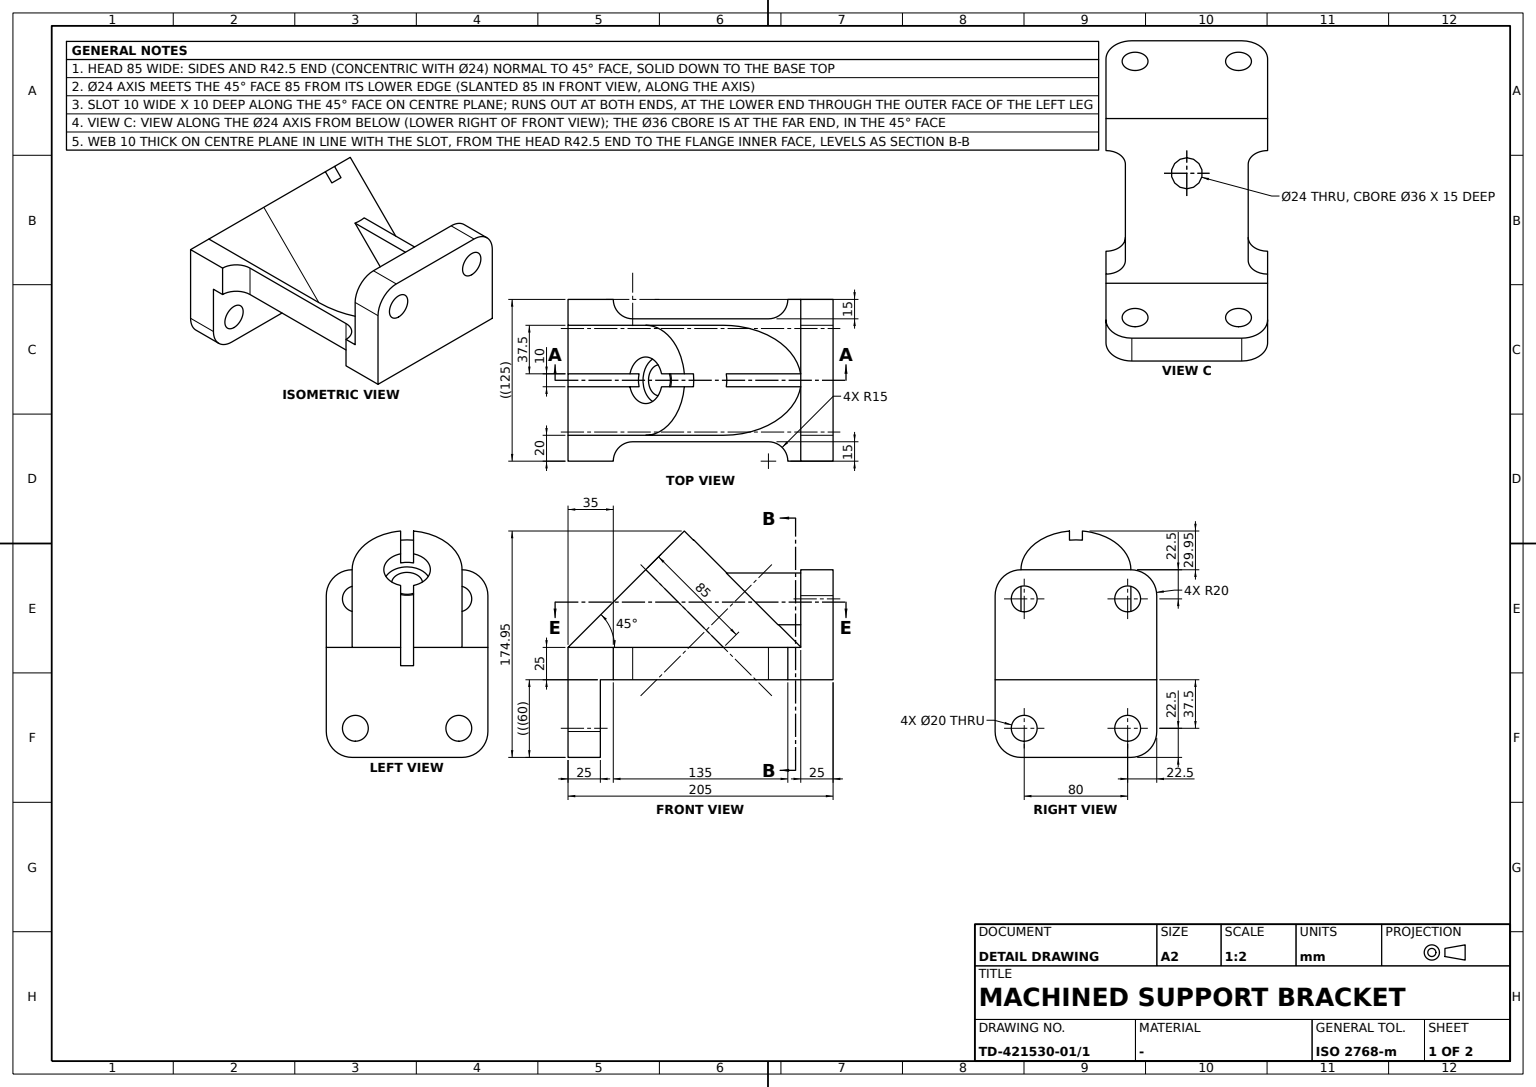
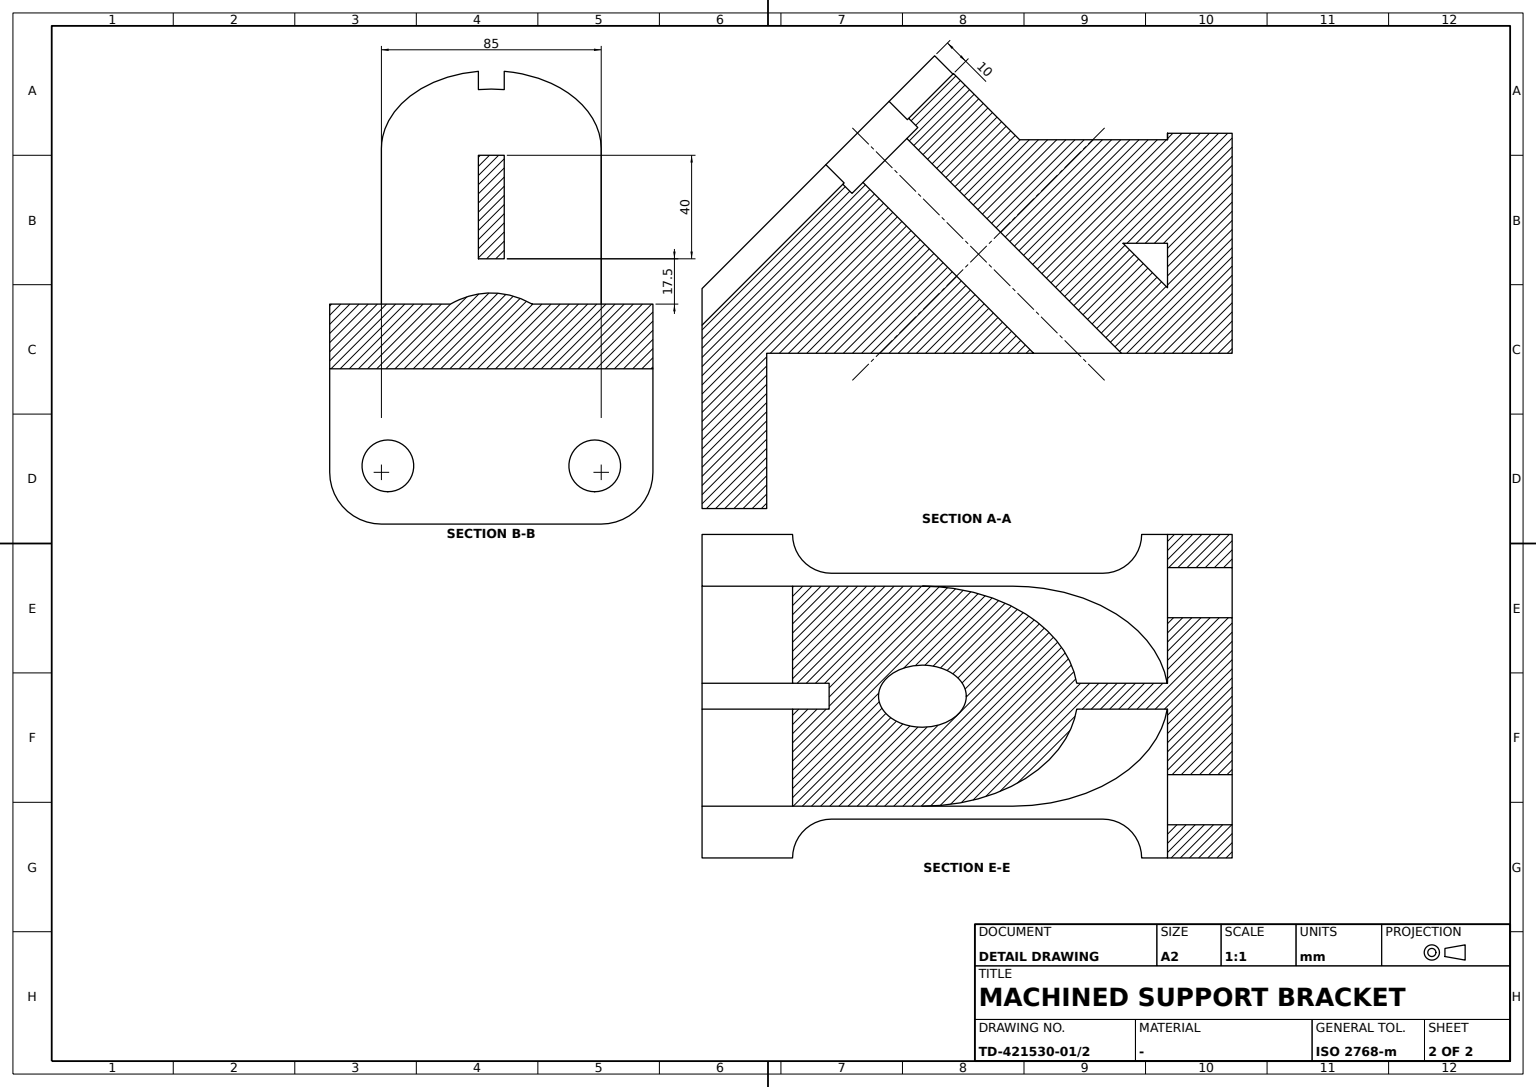
solid
v1 (0,59.678716,-12.5)
e1 v1 v1 ELLIPSE(AX(P(0,42.708153,-12.5),D(0,0,1),D(0,1,0)),16.970563,12) rev
v2 (0,-23.304041,70.482756)
e2 v2 v2 CIRCLE(AX(P(0,-31.789322,61.997475),D(0,0.707106781,-0.707106781),D(0,0.707106781,0.707106781)),12)
face CYL(AX(P(0,-42.325213,72.533366),D(0,0.707106781,-0.707106781),D(1,0,0)),12) rev [e1] [-e2]
v3 (5,77.5,30)
v4 (-5,77.5,30)
e3 v3 v4 LINE
v5 (5,59.894835,30)
e4 v3 v5 LINE
v6 (-5,59.894835,30)
e5 v5 v6 ELLIPSE(AX(P(0,0.208153,30),D(0,0,1),D(0,1,0)),60.104076,42.5)
e6 v4 v6 LINE
face PLANE(AX(P(5,77.5,30),D(0,0,1),D(-1,0,0))) rev [-e3 e4 e5 -e6]
v7 (62.5,67.5,12.5)
v8 (47.5,52.5,12.5)
e7 v7 v8 CIRCLE(AX(P(62.5,52.5,12.5),D(0,0,1),D(1,0,0)),15)
v9 (62.5,77.5,12.5)
e8 v7 v9 LINE
v10 (4.326373,77.5,12.5)
e9 v9 v10 LINE
v11 (42.5,17.708153,12.5)
e10 v11 v10 ELLIPSE(AX(P(0,17.708153,12.5),D(0,0,1),D(0,1,0)),60.104076,42.5)
v12 (42.5,-102.5,12.5)
e11 v12 v11 LINE
v13 (62.5,-102.5,12.5)
e12 v13 v12 LINE
v14 (62.5,-67.5,12.5)
e13 v13 v14 LINE
v15 (47.5,-52.5,12.5)
e14 v15 v14 CIRCLE(AX(P(62.5,-52.5,12.5),D(0,0,1),D(1,0,0)),15)
e15 v8 v15 LINE
face PLANE(AX(P(0,0,12.5),D(0,0,1),D(1,0,0))) [-e7 e8 e9 -e10 -e11 -e12 e13 -e14 -e15]
v16 (-47.5,52.5,-12.5)
v17 (-47.5,52.5,12.5)
e16 v16 v17 LINE
v18 (-62.5,67.5,12.5)
e17 v17 v18 CIRCLE(AX(P(-62.5,52.5,12.5),D(0,0,1),D(1,0,0)),15)
v19 (-62.5,67.5,-12.5)
e18 v19 v18 LINE
e19 v16 v19 CIRCLE(AX(P(-62.5,52.5,-12.5),D(0,0,1),D(1,0,0)),15)
face CYL(AX(P(-62.5,52.5,0),D(0,0,1),D(1,0,0)),15) rev [e16 e17 -e18 -e19]
v20 (47.5,52.5,-12.5)
e20 v20 v8 LINE
v21 (62.5,67.5,-12.5)
e21 v21 v20 CIRCLE(AX(P(62.5,52.5,-12.5),D(0,0,1),D(1,0,0)),15)
e22 v21 v7 LINE
face CYL(AX(P(62.5,52.5,0),D(0,0,1),D(1,0,0)),15) rev [e7 -e20 -e21 e22]
v22 (-40,102.5,40)
e23 v22 v22 CIRCLE(AX(P(-40,102.5,50),D(0,-1,0),D(0,0,-1)),10)
v23 (-62.5,102.5,-12.5)
v24 (-62.5,102.5,52.5)
e24 v23 v24 LINE
v25 (-42.5,102.5,72.5)
e25 v25 v24 CIRCLE(AX(P(-42.5,102.5,52.5),D(0,-1,0),D(0,0,-1)),20)
v26 (42.5,102.5,72.5)
e26 v25 v26 LINE
v27 (62.5,102.5,52.5)
e27 v27 v26 CIRCLE(AX(P(42.5,102.5,52.5),D(0,-1,0),D(0,0,-1)),20)
v28 (62.5,102.5,-12.5)
e28 v28 v27 LINE
e29 v23 v28 LINE
v29 (40,102.5,40)
e30 v29 v29 CIRCLE(AX(P(40,102.5,50),D(0,-1,0),D(0,0,-1)),10)
face PLANE(AX(P(-62.5,102.5,0),D(0,-1,0),D(1,0,0))) rev [e23] [e24 -e25 e26 -e27 -e28 -e29] [e30]
v30 (40,-77.5,-60)
e31 v30 v30 CIRCLE(AX(P(40,-77.5,-50),D(0,-1,0),D(0,0,-1)),10)
v31 (40,-102.5,-40)
e32 v31 v31 CIRCLE(AX(P(40,-102.5,-50),D(0,1,0),D(0,0,1)),10)
face CYL(AX(P(40,0,-50),D(0,1,0),D(-1,0,0)),10) rev [-e31] [-e32]
v32 (5,-5.481515,95.37635)
v33 (5,-23.097837,77.760028)
e33 v32 v33 LINE
v34 (-5,-5.481515,95.37635)
e34 v32 v34 CIRCLE(AX(P(0,-35.324856,65.533009),D(0,-0.707106781,0.707106781),D(0,-0.707106781,-0.707106781)),42.5)
v35 (-5,-23.097837,77.760028)
e35 v35 v34 LINE
e36 v33 v35 CIRCLE(AX(P(0,-35.324856,65.533009),D(0,-0.707106781,0.707106781),D(0,-0.707106781,-0.707106781)),18)
face PLANE(AX(P(0,-50.428932,50.428932),D(0,-0.707106781,0.707106781),D(1,0,0))) [-e33 e34 -e35 -e36]
v36 (0,-19.0614,74.725397)
e37 v36 v36 CIRCLE(AX(P(0,-31.789322,61.997475),D(0,0.707106781,-0.707106781),D(0,0.707106781,0.707106781)),18)
face PLANE(AX(P(12,-31.789322,61.997475),D(0,0.707106781,-0.707106781),D(1,0,0))) rev [-e37] [e2]
v37 (-5,19.894835,70)
v38 (5,19.894835,70)
e38 v37 v38 ELLIPSE(AX(P(0,-39.791847,70),D(0,0,-1),D(0,1,0)),60.104076,42.5)
e39 v6 v37 LINE
e40 v5 v38 LINE
v39 (5,-12.552583,102.447417)
e41 v39 v32 LINE
v40 (42.5,-42.395924,72.604076)
e42 v39 v40 CIRCLE(AX(P(0,-42.395924,72.604076),D(0,0.707106781,-0.707106781),D(0,0.707106781,0.707106781)),42.5)
e43 v40 v11 LINE
v41 (-4.326373,77.5,12.5)
e44 v10 v41 ELLIPSE(AX(P(0,77.5,-47.291847),D(0,1,0),D(0,0,-1)),60.104076,42.5) rev
v42 (-42.5,17.708153,12.5)
e45 v41 v42 ELLIPSE(AX(P(0,17.708153,12.5),D(0,0,1),D(0,1,0)),60.104076,42.5)
v43 (-42.5,-42.395924,72.604076)
e46 v43 v42 LINE
v44 (-5,-12.552583,102.447417)
e47 v43 v44 CIRCLE(AX(P(0,-42.395924,72.604076),D(0,0.707106781,-0.707106781),D(0,0.707106781,0.707106781)),42.5)
e48 v44 v34 LINE
face CYL(AX(P(0,75.695687,-45.487534),D(0,0.707106781,-0.707106781),D(-1,0,0)),42.5) [-e38 -e39 -e5 e40] [-e34 -e41 e42 e43 e10 e44 e45 -e46 e47 e48]
e49 v12 v40 LINE
face PLANE(AX(P(42.5,-102.5,12.5),D(-1,0,0),D(0,0.707106781,0.707106781))) rev [e11 -e43 -e49]
v45 (-42.5,-102.5,12.5)
v46 (-62.5,-102.5,12.5)
e50 v45 v46 LINE
e51 v45 v42 LINE
v47 (-62.5,77.5,12.5)
e52 v41 v47 LINE
e53 v47 v18 LINE
v48 (-47.5,-52.5,12.5)
e54 v17 v48 LINE
v49 (-62.5,-67.5,12.5)
e55 v49 v48 CIRCLE(AX(P(-62.5,-52.5,12.5),D(0,0,1),D(1,0,0)),15)
e56 v49 v46 LINE
face PLANE(AX(P(0,0,12.5),D(0,0,1),D(1,0,0))) [-e50 e51 -e45 e52 e53 -e17 e54 -e55 e56]
v50 (-62.5,77.5,52.5)
e57 v47 v50 LINE
e58 v50 v24 LINE
e59 v23 v19 LINE
face PLANE(AX(P(-62.5,102.5,0),D(-1,0,0),D(0,-1,0))) [e57 e58 -e24 e59 e18 -e53]
v51 (-42.5,-77.5,-72.5)
v52 (-42.5,-102.5,-72.5)
e60 v51 v52 LINE
v53 (-62.5,-102.5,-52.5)
e61 v52 v53 CIRCLE(AX(P(-42.5,-102.5,-52.5),D(0,1,0),D(0,0,1)),20)
v54 (-62.5,-77.5,-52.5)
e62 v54 v53 LINE
e63 v54 v51 CIRCLE(AX(P(-42.5,-77.5,-52.5),D(0,-1,0),D(0,0,-1)),20)
face CYL(AX(P(-42.5,-85,-52.5),D(0,-1,0),D(-1,0,0)),20) [e60 e61 -e62 e63]
e64 v21 v28 LINE
v55 (47.5,-52.5,-12.5)
e65 v20 v55 LINE
v56 (62.5,-67.5,-12.5)
e66 v55 v56 CIRCLE(AX(P(62.5,-52.5,-12.5),D(0,0,1),D(1,0,0)),15)
v57 (62.5,-77.5,-12.5)
e67 v57 v56 LINE
v58 (-62.5,-77.5,-12.5)
e68 v57 v58 LINE
v59 (-62.5,-67.5,-12.5)
e69 v59 v58 LINE
v60 (-47.5,-52.5,-12.5)
e70 v59 v60 CIRCLE(AX(P(-62.5,-52.5,-12.5),D(0,0,1),D(1,0,0)),15)
e71 v16 v60 LINE
face PLANE(AX(P(0,0,-12.5),D(0,0,1),D(1,0,0))) rev [-e59 e29 -e64 e21 e65 e66 -e67 e68 -e69 e70 -e71 e19] [-e1]
v61 (42.5,77.5,72.5)
v62 (-42.5,77.5,72.5)
e72 v61 v62 LINE
e73 v61 v26 LINE
e74 v62 v25 LINE
face PLANE(AX(P(0,0,72.5),D(0,0,1),D(1,0,0))) [-e72 e73 -e26 -e74]
v63 (-5,77.5,70)
e75 v63 v37 LINE
e76 v4 v63 LINE
face PLANE(AX(P(-5,-114.068542,0.931458),D(-1,0,0),D(0,0.707106781,0.707106781))) [e6 e39 -e75 -e76]
v64 (42.5,-77.5,-72.5)
v65 (42.5,-102.5,-72.5)
e77 v64 v65 LINE
v66 (62.5,-77.5,-52.5)
e78 v64 v66 CIRCLE(AX(P(42.5,-77.5,-52.5),D(0,-1,0),D(0,0,-1)),20)
v67 (62.5,-102.5,-52.5)
e79 v66 v67 LINE
e80 v67 v65 CIRCLE(AX(P(42.5,-102.5,-52.5),D(0,1,0),D(0,0,1)),20)
face CYL(AX(P(42.5,-85,-52.5),D(0,-1,0),D(1,0,0)),20) [-e77 e78 e79 e80]
e81 v43 v45 LINE
face PLANE(AX(P(-42.5,-42.395924,72.604076),D(1,0,0),D(0,-0.707106781,-0.707106781))) rev [-e51 -e81 e46]
e82 v53 v46 LINE
e83 v59 v49 LINE
e84 v58 v54 LINE
face PLANE(AX(P(-62.5,102.5,0),D(-1,0,0),D(0,-1,0))) [e62 e82 -e56 -e83 e69 e84]
v68 (-40,-77.5,-60)
e85 v68 v68 CIRCLE(AX(P(-40,-77.5,-50),D(0,-1,0),D(0,0,-1)),10)
e86 v64 v51 LINE
e87 v57 v66 LINE
face PLANE(AX(P(62.5,-77.5,-12.5),D(0,-1,0),D(-1,0,0))) rev [e85] [-e78 e86 -e63 -e84 -e68 e87] [e31]
v69 (5,-30.168904,84.831096)
e88 v33 v69 LINE
e89 v39 v69 LINE
face PLANE(AX(P(5,-0.931458,114.068542),D(1,0,0),D(0,-0.707106781,-0.707106781))) rev [e41 e33 e88 -e89]
v70 (-5,-102.5,-1.642136)
v71 (5,-102.5,-1.642136)
e90 v70 v71 LINE
v72 (5,-47.551875,53.305989)
e91 v72 v71 LINE
v73 (-5,-47.551875,53.305989)
e92 v73 v72 CIRCLE(AX(P(0,-35.324856,65.533009),D(0,-0.707106781,0.707106781),D(0,-0.707106781,-0.707106781)),18)
e93 v70 v73 LINE
face PLANE(AX(P(0,-50.428932,50.428932),D(0,-0.707106781,0.707106781),D(1,0,0))) [e90 -e91 -e92 -e93]
e94 v60 v48 LINE
face CYL(AX(P(-62.5,-52.5,0),D(0,0,1),D(1,0,0)),15) rev [e83 e55 -e94 -e70]
v74 (5,-54.622943,60.377057)
e95 v69 v74 CIRCLE(AX(P(0,-42.395924,72.604076),D(0,0.707106781,-0.707106781),D(0,0.707106781,0.707106781)),18)
v75 (5,-102.5,12.5)
e96 v74 v75 LINE
e97 v75 v12 LINE
face PLANE(AX(P(0,-57.5,57.5),D(0,0.707106781,-0.707106781),D(-1,0,0))) rev [e89 e95 e96 e97 e49 -e42]
e98 v74 v72 LINE
e99 v75 v71 LINE
face PLANE(AX(P(5,-0.931458,114.068542),D(1,0,0),D(0,-0.707106781,-0.707106781))) rev [e98 e91 -e99 -e96]
e100 v52 v65 LINE
face PLANE(AX(P(0,0,-72.5),D(0,0,-1),D(1,0,0))) [-e86 e77 -e100 -e60]
v76 (-5,-30.168904,84.831096)
e101 v76 v35 LINE
v77 (-5,-54.622943,60.377057)
e102 v77 v76 CIRCLE(AX(P(0,-42.395924,72.604076),D(0,0.707106781,-0.707106781),D(0,0.707106781,0.707106781)),18)
e103 v73 v77 LINE
face CYL(AX(P(0,-42.325213,72.533366),D(0,0.707106781,-0.707106781),D(1,0,0)),18) rev [e92 -e98 -e95 -e88 e36 -e101 -e102 -e103] [e37]
v78 (5,77.5,70)
e104 v78 v38 LINE
e105 v63 v78 LINE
face PLANE(AX(P(-5,77.5,70),D(0,0,-1),D(1,0,0))) rev [e75 e38 -e104 -e105]
v79 (62.5,77.5,52.5)
e106 v61 v79 CIRCLE(AX(P(42.5,77.5,52.5),D(0,1,0),D(0,0,1)),20)
e107 v79 v27 LINE
face CYL(AX(P(42.5,85,52.5),D(0,1,0),D(1,0,0)),20) [-e73 e106 e107 e27]
e108 v50 v62 CIRCLE(AX(P(-42.5,77.5,52.5),D(0,1,0),D(0,0,1)),20)
e109 v9 v79 LINE
v80 (40,77.5,60)
e110 v80 v80 CIRCLE(AX(P(40,77.5,50),D(0,1,0),D(0,0,1)),10)
v81 (-40,77.5,60)
e111 v81 v81 CIRCLE(AX(P(-40,77.5,50),D(0,1,0),D(0,0,1)),10)
e112 v78 v3 LINE
face PLANE(AX(P(62.5,77.5,12.5),D(0,1,0),D(-1,0,0))) rev [-e106 e72 -e108 -e57 -e52 -e44 -e9 e109] [e110] [e111] [e76 e105 e112 e3]
v82 (-5,-102.5,12.5)
e113 v82 v77 LINE
e114 v82 v70 LINE
face PLANE(AX(P(-5,-114.068542,0.931458),D(-1,0,0),D(0,0.707106781,0.707106781))) rev [-e113 e114 e93 e103]
face PLANE(AX(P(5,-0.931458,114.068542),D(1,0,0),D(0,-0.707106781,-0.707106781))) [-e112 e104 -e40 -e4]
e115 v45 v82 LINE
e116 v67 v13 LINE
v83 (-40,-102.5,-40)
e117 v83 v83 CIRCLE(AX(P(-40,-102.5,-50),D(0,1,0),D(0,0,1)),10)
face PLANE(AX(P(62.5,-102.5,0),D(0,1,0),D(-1,0,0))) rev [e12 -e97 e99 -e90 -e114 -e115 e50 -e82 -e61 e100 -e80 e116] [e32] [e117]
e118 v76 v44 LINE
face PLANE(AX(P(0,-57.5,57.5),D(0,0.707106781,-0.707106781),D(-1,0,0))) rev [e115 e113 e102 e118 -e47 e81]
face PLANE(AX(P(-5,-114.068542,0.931458),D(-1,0,0),D(0,0.707106781,0.707106781))) rev [-e118 e101 e35 -e48]
face CYL(AX(P(-40,0,-50),D(0,1,0),D(-1,0,0)),10) rev [-e117] [-e85]
face CYL(AX(P(-40,0,50),D(0,1,0),D(-1,0,0)),10) rev [-e23] [-e111]
e119 v55 v15 LINE
face PLANE(AX(P(47.5,52.5,0),D(-1,0,0),D(0,-1,0))) rev [e20 e15 -e119 -e65]
face PLANE(AX(P(62.5,-102.5,0),D(1,0,0),D(0,1,0))) [-e107 -e109 -e8 -e22 e64 e28]
face CYL(AX(P(-42.5,85,52.5),D(0,1,0),D(-1,0,0)),20) [e74 e25 -e58 e108]
face PLANE(AX(P(-47.5,52.5,0),D(-1,0,0),D(0,-1,0))) [-e54 -e16 e71 e94]
e120 v56 v14 LINE
face PLANE(AX(P(62.5,-102.5,0),D(1,0,0),D(0,1,0))) [e120 -e13 -e116 -e79 -e87 e67]
face CYL(AX(P(40,0,50),D(0,1,0),D(-1,0,0)),10) rev [-e110] [-e30]
face CYL(AX(P(62.5,-52.5,0),D(0,0,1),D(1,0,0)),15) rev [-e120 -e66 e119 e14]
